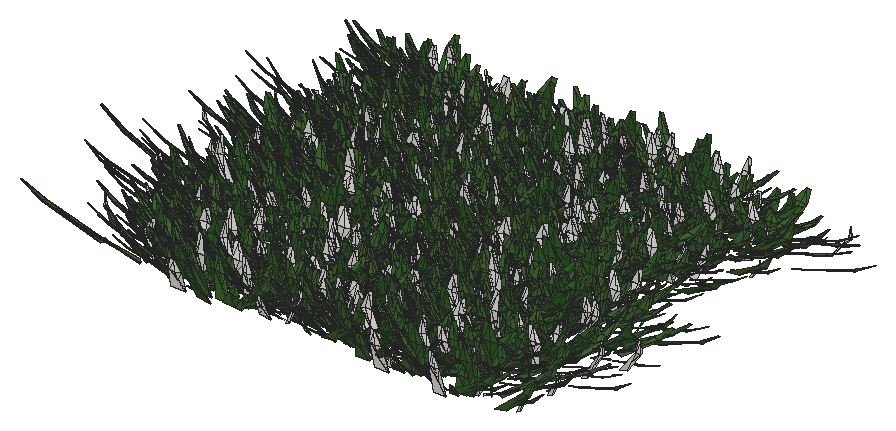
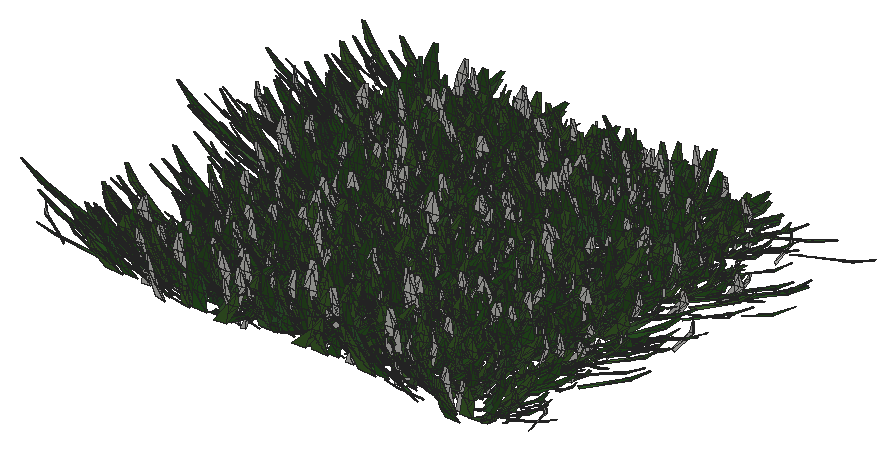
# SketchUp Ruby script. Lengths in inches.
U = 1.inch
M = Sketchup.active_model
def pt(a) = Geom::Point3d.new(a.map { |v| v * U })
def face(e, loops, mat)
  f = e.add_face(loops[0].map { |a| pt(a) })
  loops[1..].each { |l| e.add_face(l.map { |a| pt(a) }).erase! }
  f.material = f.back_material = mat if mat
  f
end
# faces: each face lists its corners as indices into pts; further lists are holes
def faces(e, pts, list, mat = nil) = list.each { |f| face(e, (f[0].is_a?(Array) ? f : [f]).map { |l| l.map { |i| pts[i] } }, mat) }
# xy, xz, yz: faces in a plane at the given z, y or x. An outline is a flat list of corners, or four numbers for a rectangle; further outlines are holes
def ring(l) = l.size == 4 ? [[l[0], l[1]], [l[2], l[1]], [l[2], l[3]], [l[0], l[3]]] : l.each_slice(2).to_a
def flat(e, list, mat, &to3) = list.each { |f| face(e, (f[0].is_a?(Array) ? f : [f]).map { |l| ring(l).map { |u, v| to3.(u, v) } }, mat) }
def xy(e, z, list, mat = nil) = flat(e, list, mat) { |x, y| [x, y, z] }
def xz(e, y, list, mat = nil) = flat(e, list, mat) { |x, z| [x, y, z] }
def yz(e, x, list, mat = nil) = flat(e, list, mat) { |y, z| [x, y, z] }
def lines(e, pts, list) = list.each { |a, b| e.add_line(pt(pts[a]), pt(pts[b])) }
# prism: a flat outline (further loops are holes) pulled along v
def prism(e, loops, v, mat = nil)
  f = face(e, loops, mat); d = Geom::Vector3d.new(v.map { |x| x * U })
  f.pushpull(f.normal.samedirection?(d) ? d.length : -d.length)
end
def box(e, o, s, mat = nil) = prism(e, [[o, [o[0] + s[0], o[1], o[2]], [o[0] + s[0], o[1] + s[1], o[2]], [o[0], o[1] + s[1], o[2]]]], [0, 0, s[2]], mat)
def at(x, y, z, deg = 0) = Geom::Transformation.translation(pt([x, y, z])) * Geom::Transformation.rotation(ORIGIN, Z_AXIS, deg.degrees)
def axes(o, x, y, z) = Geom::Transformation.new([*x, 0, *y, 0, *z, 0, *pt(o).to_a, 1])
def part(name) = M.definitions.add(name)
# library, detail: a bought-in or finely detailed component or shape, given as its bounding box
def library(name, o, s) = part(name).tap { |d| box(d.entities, o, s) }
def detail(e, o, s) = box(e.add_group.entities, o, s)
def put(e, d, t, mat = nil) = e.add_instance(d, t).tap { |i| i.material = mat if mat }
def group(e, t, mat = nil) = e.add_group.tap { |g| g.transformation = t; g.material = mat if mat }.entities
root = M.entities
M.materials.add("Material10").color = [48, 100, 38]
M.materials.add("Material3").color = [68, 110, 58]
M.materials.add("Material4").color = [48, 90, 38]
M.materials.add("Material5").color = [68, 110, 48]
M.materials.add("Material6").color = [48, 90, 48]
M.materials.add("Material7").color = [58, 110, 58]
M.materials.add("Material8").color = [58, 90, 38]
M.materials.add("Material9").color = [68, 100, 58]
c1 = part("grass00")
p = [[-0.6875,0.15,0],[-0.56,0.08,5.52],[-0.04,0.03,2.76],[0.48,-0.02,0],[0.35,-0.02,5.52],[-0.1,-0.14,5.52],
  [-0.12,0.65,8.37],[-0.42,0.65,8.37]]
faces(c1.entities,p,[[0,1,2,3],[3,2,4],[1,5,2],[5,4,2],[1,6,5],[4,5,6],[7,6,1]])
c2 = part("Group16\#1")
put(c2.entities,c1,axes([1.44,-0.61,-0.01],[0.05352,0.12609,0],[-0.10704,0.04543,0.07239],[0.06664,-0.02828,0.11628]),"Material6")
put(c2.entities,c1,axes([0.76,-0.15,-0.01],[0.04676,0.24062,0],[-0.23162,0.04501,0.06642],[0.0652,-0.01267,0.23595]),"Material3")
put(c2.entities,c1,axes([0.79,0.01,-0.01],[-0.00606,0.34651,0],[-0.34381,-0.00602,0.0432],[0.04319,0.00076,0.34386]))
put(c2.entities,c1,axes([1,0.23,-0.01],[-0.07192,0.31144,0],[-0.28722,-0.06632,0.1236],[0.12043,0.02781,0.29478]),"Material5")
put(c2.entities,c1,axes([1.66,0.77,-0.01],[-0.13828,0.29651,0],[-0.21551,-0.1005,0.22471],[0.20365,0.09498,0.23779]),"Material10")
put(c2.entities,c1,axes([0.6875,0.52,-0.01],[-0.18126,0.24051,0],[-0.22746,-0.17142,0.09788],[0.07817,0.05891,0.28481]),"Material5")
put(c2.entities,c1,axes([0.68,0.78,-0.01],[-0.215,0.18688,0],[-0.12385,-0.14248,0.21334],[0.13995,0.16101,0.18878]),"Material3")
put(c2.entities,c1,axes([0.56,1,-0.01],[-0.13756,0.07624,0],[-0.06159,-0.11112,0.0927],[0.04494,0.08108,0.12705]),"Material5")
put(c2.entities,c1,axes([0.2,0.64,-0.01],[-0.23729,0.07254,0],[-0.05711,-0.18681,0.153],[0.04473,0.14632,0.19535]),"Material10")
put(c2.entities,c1,axes([0.0625,0.72,-0.01],[-0.28874,0.02525,0],[-0.02179,-0.24916,0.14647],[0.01276,0.14591,0.25012]),"Material3")
put(c2.entities,c1,axes([-0.08,0.62,-0.01],[-0.34089,-0.04187,0],[0.03255,-0.26504,0.216],[-0.02633,0.21439,0.26703]),"Material10")
put(c2.entities,c1,axes([-0.34,0.98,-0.01],[-0.14314,-0.0493,0],[0.04397,-0.12769,0.06843],[-0.02228,0.0647,0.13505]),"Material10")
put(c2.entities,c1,axes([-0.87,1.45,-0.01],[-0.23488,-0.14114,0],[0.13761,-0.22901,0.06087],[-0.03135,0.05217,0.26717]))
put(c2.entities,c1,axes([-0.72,0.77,-0.01],[-0.14208,-0.13251,0],[0.07209,-0.0773,0.16301],[-0.11118,0.11922,0.1057]),"Material10")
put(c2.entities,c1,axes([-0.62,0.43,-0.01],[-0.14845,-0.21203,0],[0.18654,-0.13061,0.12304],[-0.10079,0.07057,0.22772]),"Material3")
put(c2.entities,c1,axes([-0.68,0.29,-0.01],[-0.13639,-0.32136,0],[0.31723,-0.13464,0.05579],[-0.05136,0.0218,0.34462]),"Material4")
put(c2.entities,c1,axes([-0.64,0.125,-0.01],[-0.0458,-0.23569,0],[0.22124,-0.043,0.08276],[-0.08124,0.01579,0.22538]),"Material7")
put(c2.entities,c1,axes([-1.6,-0.03,-0.01],[0.00576,-0.32897,0],[0.27526,0.00482,0.18018],[-0.18015,-0.00315,0.2753]),"Material5")
put(c2.entities,c1,axes([-1.36,-0.31,-0.01],[0.05718,-0.24765,0],[0.18172,0.04196,0.17267],[-0.16825,-0.03885,0.1865]),"Material10")
put(c2.entities,c1,axes([-1.54,-0.72,-0.01],[0.06537,-0.14017,0],[0.13555,0.06321,0.03939],[-0.0357,-0.01665,0.14956]))
put(c2.entities,c1,axes([-1.19,-0.9,-0.01],[0.09597,-0.12735,0],[0.11214,0.08451,0.07557],[-0.06035,-0.04548,0.14042]),"Material9")
put(c2.entities,c1,axes([-0.47,-0.54,-0.01],[0.11588,-0.10072,0],[0.0618,0.0711,0.12124],[-0.07953,-0.0915,0.0942]))
put(c2.entities,c1,axes([-0.47,-0.84,-0.01],[0.11927,-0.0661,0],[0.06603,0.11913,0.00646],[-0.00313,-0.00565,0.13621]),"Material5")
put(c2.entities,c1,axes([-0.38,-1.24,-0.01],[0.28037,-0.08571,0],[0.0618,0.20215,0.20315],[-0.05939,-0.19428,0.21139]),"Material9")
put(c2.entities,c1,axes([-0.06,-0.66,-0.01],[0.22719,-0.01987,0],[0.01247,0.14255,0.17758],[-0.01547,-0.17691,0.1431]),"Material8")
put(c2.entities,c1,axes([0.11,-0.89,-0.01],[0.14882,0.01828,0],[-0.01058,0.08611,0.12229],[0.01491,-0.12138,0.08676]),"Material6")
put(c2.entities,c1,axes([0.25,-0.72,-0.01],[0.20481,0.07053,0],[-0.06206,0.18022,0.10291],[0.03351,-0.0973,0.1906]),"Material6")
put(c2.entities,c1,axes([0.85,-1.42,-0.01],[0.16481,0.09904,0],[-0.09472,0.15762,0.05616],[0.02893,-0.04814,0.18389]),"Material5")
put(c2.entities,c1,axes([1.01,-1.09,-0.01],[0.21858,0.20385,0],[-0.17495,0.1876,0.15339],[0.10462,-0.11218,0.25652]),"Material10")
put(c2.entities,c1,axes([1.01,-0.71,-0.01],[0.08733,0.12473,0],[-0.06445,0.04512,0.13037],[0.1068,-0.07477,0.07867]),"Material6")
c3 = part("Group15\#1")
put(c3.entities,c2,at(0,0,0))
c4 = part("3darcstudiotree_grass00\#1")
put(c4.entities,c3,at(0,0,0))
put(root,c4,axes([124.42,82.5,7.6],[1.41495,1.18383,0],[-3.49756,0.26127,-0.01522],[-0.0888,0.00663,1.38916]))
put(root,c4,axes([126.49,54.95,7.6],[-4.73179,-0.12886,0],[0.46967,-1.07792,-0.0047],[0.00279,-0.0064,1.4854]))
put(root,c4,axes([124.78,64.93,7.6],[0.18591,1.26274,0],[-5.04075,0.04638,-0.03073],[-0.14495,0.00133,1.48809]))
put(root,c4,axes([126.5625,74.74,7.6],[-4.30621,-0.01829,0],[0.08217,-1.20899,-0.03595],[0.00336,-0.04947,1.66434]))
put(root,c4,axes([126.89,66.41,7.6],[-3.87854,-0.40989,0],[1.77421,-1.04926,-0.0473],[0.09277,-0.05486,1.43445]))
put(root,c4,axes([124.91,54.12,7.6],[4.45359,0.5299,0],[-1.68792,0.88663,-0.01473],[-0.03849,0.02022,1.49308]))
put(root,c4,axes([126.65,57.24,7.6],[-4.3672,0.54864,0],[-1.80768,-0.89932,-0.0516],[-0.17927,-0.08919,1.94674]))
put(root,c4,axes([127.23,59.97,7.6],[-4.20222,0.09704,0],[-0.34915,-0.94494,-0.04806],[-0.02957,-0.08003,1.58689]))
put(root,c4,axes([126.96,73.125,7.6],[2.2244,-0.73123,0],[4.08618,0.77689,-0.04371],[0.15259,0.02901,1.40723]))
put(root,c4,axes([128.02,79.75,7.6],[-4.09129,-0.53085,0],[1.96428,-0.94617,-0.02416],[0.06052,-0.02915,1.4491]))
put(root,c4,axes([128.07,78.01,7.6],[-3.27232,-0.38033,0],[1.61038,-0.86597,-0.04575],[0.12951,-0.06964,1.60296]))
put(root,c4,axes([126.875,69.46,7.6],[1.34498,0.85271,0],[-3.61197,0.35607,-0.04901],[-0.30956,0.03052,1.64754]))
put(root,c4,axes([128.14,51.875,7.6],[-3.74465,0.10964,0],[-0.44388,-0.94751,-0.03745],[-0.02749,-0.05868,1.50509]))
put(root,c4,axes([126.73,47.91,7.6],[0.55868,1.18187,0],[-4.38906,0.12967,-0.00527],[-0.02848,0.00084,1.50433]))
put(root,c4,axes([127.38,81.63,7.6],[3.92571,-0.06568,0],[0.27031,1.00981,-0.02393],[0.00951,0.03553,1.50627]))
put(root,c4,axes([127.24,67.3,7.6],[4.1204,0.14772,0],[-0.55424,0.96623,-0.02285],[-0.01788,0.03117,1.34478]))
put(root,c4,axes([128.85,44.9375,7.6],[-4.54837,0.61423,0],[-2.27056,-1.05085,-0.03525],[-0.07342,-0.03398,1.3087]))
put(root,c4,axes([129.04,49.74,7.6],[1.35556,-1.09662,0],[3.48641,0.26935,-0.00928],[0.07297,0.00564,1.87692]))
put(root,c4,axes([127.76,58.58,7.6],[4.58081,0.57203,0],[-2.05118,1.02662,-0.04234],[-0.09467,0.04738,1.4356]))
put(root,c4,axes([128.33,72.32,7.6],[4.09069,0.39107,0],[-1.49345,0.97637,-0.02441],[-0.06576,0.04299,1.97124]))
put(root,c4,axes([128.3,70.53,7.6],[4.67312,0.46375,0],[-1.55175,0.97728,-0.04113],[-0.07938,0.05,1.37498]))
put(root,c4,axes([128.86,76.31,7.6],[1.74991,0.88126,0],[-3.81182,0.47307,-0.01001],[-0.04959,0.00615,1.4706]))
put(root,c4,axes([130.88,63.98,7.6],[-4.64971,-0.14285,0],[0.57946,-1.17887,-0.04768],[0.02933,-0.05967,1.49744]))
put(root,c4,axes([129.26,53.72,7.6],[0.96395,1.06005,0],[-4.81113,0.27344,-0.06457],[-0.29518,0.01678,1.44574]))
put(root,c4,axes([130.38,46.22,7.6],[3.00205,-0.85659,0],[3.63036,0.7952,-0.04981],[0.2075,0.04545,1.67091]))
put(root,c4,axes([129.4,62.67,7.6],[3.43592,0.73211,0],[-2.51322,0.73719,-0.00613],[-0.02752,0.00807,1.67562]))
put(root,c4,axes([130.35,50.32,7.6],[1.74385,0.8383,0],[-3.77239,0.49046,-0.03549],[-0.18091,0.02352,1.52707]))
put(root,c4,axes([130.11,61.6,7.6],[1.69559,1.05532,0],[-4.4836,0.45024,-0.00669],[-0.03988,0.004,1.94122]))
put(root,c4,axes([133.36,44.27,7.6],[-2.1334,-0.73078,0],[3.43772,-0.62725,-0.00015],[0.00089,-0.00016,1.94435]))
put(root,c4,axes([133.04,61.22,7.6],[-0.05318,-0.92593,0],[5.00241,-0.01796,-0.06189],[0.33029,-0.00119,1.66883]))
put(root,c4,axes([133.4,80.03,7.6],[-3.23712,-0.63399,0],[2.66966,-0.85194,-0.04081],[0.13619,-0.04346,1.46417]))
put(root,c4,axes([133.35,73.37,7.6],[-4.03858,-0.16836,0],[0.61274,-0.91864,-0.01602],[0.01597,-0.02395,1.41148]))
put(root,c4,axes([134.01,81.37,7.6],[-0.4686,-0.94109,0],[4.875,-0.15171,-0.05859],[0.34766,-0.01082,1.83593]))
put(root,c4,axes([134.38,66.01,7.6],[-4.976,0.12548,0],[-0.39366,-0.97566,-0.00469],[-0.00376,-0.00932,1.96044]))
put(root,c4,axes([134.65,67.66,7.6],[-3.93213,0.25374,0],[-1.01516,-0.98322,-0.03018],[-0.05893,-0.05707,1.98332]))
put(root,c4,axes([135.21,77.64,7.6],[-3.81287,-0.39073,0],[1.76767,-1.0781,-0.01809],[0.03493,-0.0213,1.4829]))
put(root,c4,axes([134.63,76.28,7.6],[1.16902,-1.01976,0],[4.12301,0.2954,-0.03571],[0.25113,0.01799,1.9611]))
put(root,c4,axes([134.76,46.48,7.6],[-3.57612,0.46,0],[-1.68045,-0.8165,-0.01759],[-0.06739,-0.03274,1.92222]))
put(root,c4,axes([134.52,55.21,7.6],[2.75353,-0.91552,0],[4.13951,0.77813,-0.05965],[0.29097,0.05469,1.97549]))
put(root,c4,axes([133.67,70.53,7.6],[4.41787,0.20597,0],[-0.82473,1.10563,-0.00417],[-0.0051,0.00683,1.87295]))
put(root,c4,axes([135.39,56.4,7.6],[-0.77256,-1.09422,0],[3.72876,-0.16454,-0.01992],[0.13289,-0.00586,1.60321]))
put(root,c4,axes([133.66,52.31,7.6],[4.90123,0.13236,0],[-0.55386,1.28181,-0.03307],[-0.01756,0.04064,1.59331]))
put(root,c4,axes([134.13,63.08,7.6],[0.63816,1.22279,0],[-3.70201,0.12075,-0.03746],[-0.26805,0.00874,1.68385]))
put(root,c4,axes([134.88,50.37,7.6],[-3.38877,0.51557,0],[-2.38455,-0.97958,-0.01391],[-0.04361,-0.01791,1.7292]))
put(root,c4,axes([135.11,53.53,7.6],[2.69835,-0.96968,0],[3.12111,0.54282,-0.02795],[0.17981,0.03127,1.86246]))
put(root,c4,axes([134.76,69.01,7.6],[-2.15572,1.01928,0],[-4.46043,-0.5896,-0.01892],[-0.07769,-0.01027,1.46501]))
put(root,c4,axes([136.66,75.07,7.6],[-3.178,-0.72198,0],[3.25819,-0.89636,-0.02206],[0.07961,-0.0219,1.62457]))
put(root,c4,axes([135,58.75,7.6],[-2.01821,1.07087,0],[-4.04462,-0.47641,-0.00165],[-0.00796,-0.00094,1.48801]))
put(root,c4,axes([136.75,47.43,7.6],[-5.04293,-0.12413,0],[0.46059,-1.16949,-0.00134],[0.0006,-0.00152,1.33719]))
put(root,c4,axes([134.69,72.55,7.6],[1.81913,1.13072,0],[-4.24624,0.42697,-0.0015],[-0.00751,0.00076,1.54039]))
put(root,c4,axes([136.29,49.35,7.6],[2.93485,-0.98597,0],[3.93521,0.7321,-0.05496],[0.20354,0.03787,1.41537]))
put(root,c4,axes([136.5,59.75,7.6],[0.69977,0.95429,0],[-4.68091,0.21453,-0.00804],[-0.04724,0.00217,1.77733]))
put(root,c4,axes([136.77,64.87,7.6],[2.05265,1.08844,0],[-3.86298,0.45532,-0.03917],[-0.23834,0.02809,1.79585]))
put(root,c4,axes([139.52,47.65,7.6],[-1.12524,-0.96886,0],[3.74948,-0.27217,-0.00444],[0.03259,-0.00237,1.86591]))
put(root,c4,axes([138.9,61.27,7.6],[1.4605,-0.95002,0],[3.8779,0.3726,-0.03841],[0.24153,0.02321,1.74904]))
put(root,c4,axes([139.41,67.22,7.6],[-2.14754,-0.73736,0],[3.76224,-0.68483,-0.06067],[0.30518,-0.05555,1.80988]))
put(root,c4,axes([139.29,50.73,7.6],[-3.33972,0.41247,0],[-1.92358,-0.97344,-0.03032],[-0.07425,-0.03758,1.50108]))
put(root,c4,axes([139.27,72.47,7.6],[3.71164,-0.61185,0],[2.58785,0.98115,-0.02666],[0.07433,0.02818,1.48784]))
put(root,c4,axes([140.375,81.02,7.6],[0.28174,-1.01382,0],[4.36389,0.07579,-0.0172],[0.10528,0.00183,1.67763]))
put(root,c4,axes([139.93,45.37,7.6],[-2.86097,0.86073,0],[-3.01972,-0.62732,-0.04997],[-0.22994,-0.04777,1.46822]))
put(root,c4,axes([141.125,71.12,7.6],[-4.12883,-0.65967,0],[2.58219,-1.01011,-0.05584],[0.19452,-0.07609,1.93872]))
put(root,c4,axes([139.63,49.74,7.6],[-0.2845,0.94758,0],[-4.0362,-0.07574,-0.02554],[-0.16533,-0.0031,1.64241]))
put(root,c4,axes([141.5625,53.39,7.6],[-4.76231,0.21357,0],[-0.8747,-1.21904,-0.00093],[-0.00084,-0.00117,1.58752]))
put(root,c4,axes([140.26,46.6,7.6],[4.17112,0.04454,0],[-0.19892,1.16431,-0.01987],[-0.00428,0.02505,1.47043]))
put(root,c4,axes([140.29,55.31,7.6],[4.56851,-0.0546,0],[0.17436,0.91177,-0.03217],[0.01167,0.06102,1.73328]))
put(root,c4,axes([140.5,56.74,7.6],[4.23657,-0.2376,0],[0.80233,0.89415,-0.00297],[0.00478,0.00533,1.68702]))
put(root,c4,axes([142.35,78.12,7.6],[-3.12199,-0.46434,0],[2.64637,-1.11204,-0.00321],[0.00751,-0.00316,1.48019]))
put(root,c4,axes([141.49,73.17,7.6],[-3.87477,0.75183,0],[-2.84001,-0.9148,-0.03049],[-0.11215,-0.03613,1.73706]))
put(root,c4,axes([140.73,63.55,7.6],[3.58042,0.48605,0],[-1.82681,0.84106,-0.03457],[-0.13256,0.06103,1.92264]))
put(root,c4,axes([141.78,76.84,7.6],[2.19573,-0.79563,0],[3.28578,0.56674,-0.0362],[0.23043,0.03975,1.92943]))
put(root,c4,axes([141.35,52.67,7.6],[-1.60767,1.01804,0],[-4.53552,-0.44765,-0.02576],[-0.12044,-0.01189,1.53201]))
put(root,c4,axes([141.4375,58.17,7.6],[4.66104,-0.01291,0],[0.04336,0.97863,-0.01976],[0.00122,0.02762,1.36845]))
put(root,c4,axes([141.69,65.9375,7.6],[2.73136,0.67519,0],[-2.53096,0.63991,-0.02576],[-0.15171,0.03836,1.88472]))
put(root,c4,axes([141.8,68.65,7.6],[4.8227,0.33397,0],[-1.37587,1.24178,-0.02222],[-0.03562,0.03215,1.93436]))
put(root,c4,axes([142.17,79.72,7.6],[2.66703,0.73786,0],[-3.13866,0.70905,-0.0306],[-0.16013,0.03617,1.86488]))
put(root,c4,axes([143.03,59.4375,7.6],[-2.52556,0.85651,0],[-3.11909,-0.57482,-0.0238],[-0.1265,-0.02331,1.59896]))
put(root,c4,axes([142.32,75.5625,7.6],[1.56451,1.00298,0],[-4.78607,0.4666,-0.01645],[-0.08409,0.0082,1.76201]))
put(root,c4,axes([142.62,65.03,7.6],[1.42494,0.93436,0],[-3.83119,0.36517,-0.01397],[-0.07753,0.00739,1.52193]))
put(root,c4,axes([145.43,46.8125,7.6],[-3.14311,-1.03345,0],[3.53925,-0.67276,-0.02],[0.10195,-0.01938,1.779]))
put(root,c4,axes([145.19,47.78,7.6],[-0.38253,-1.25706,0],[5.07372,-0.0965,-0.05882],[0.29497,-0.00561,1.5994]))
put(root,c4,axes([145.6,55.89,7.6],[-3.9211,-0.27648,0],[1.04934,-0.93013,-0.015],[0.02202,-0.01952,1.30652]))
put(root,c4,axes([144.72,78.3125,7.6],[-0.95414,1.15068,0],[-4.04773,-0.20977,-0.02464],[-0.16776,-0.00869,1.79662]))
put(root,c4,axes([145.44,49.37,7.6],[-3.41535,0.94101,0],[-3.19182,-0.72403,-0.0082],[-0.03901,-0.00885,1.73071]))
put(root,c4,axes([145.14,77.02,7.6],[-0.26244,0.97433,0],[-4.33641,-0.073,-0.04305],[-0.28268,-0.00476,1.78778]))
put(root,c4,axes([146.28,65.52,7.6],[-4.734,0.44651,0],[-1.80443,-1.19569,-0.03096],[-0.06152,-0.04076,1.79846]))
put(root,c4,axes([146.89,54.35,7.6],[-3.54413,-0.35283,0],[1.88693,-1.18461,-0.01803],[0.03799,-0.02385,1.81493]))
put(root,c4,axes([145.7,62.8125,7.6],[-1.93923,0.80033,0],[-4.36084,-0.6604,-0.05645],[-0.30002,-0.04543,1.97994]))
put(root,c4,axes([147.17,74.11,7.6],[-1.73824,-0.83269,0],[3.93121,-0.5129,-0.00435],[0.02089,-0.00273,1.50222]))
put(root,c4,axes([145.54,61.65,7.6],[3.26249,0.60372,0],[-2.60827,0.88094,-0.05487],[-0.17274,0.05834,1.44987]))
put(root,c4,axes([145.65,79.57,7.6],[0.73959,1.18717,0],[-3.65318,0.14224,-0.00889],[-0.05312,0.00207,1.39664]))
put(root,c4,axes([146.51,81.39,7.6],[2.83501,-0.87969,0],[3.07253,0.61887,-0.02709],[0.15503,0.03123,1.8123]))
put(root,c4,axes([145.54,70.86,7.6],[4.22317,0.50582,0],[-2.02967,1.05913,-0.04599],[-0.0924,0.04822,1.36526]))
put(root,c4,axes([147.79,74.82,7.6],[-3.49567,-0.41418,0],[1.84622,-0.97387,-0.03887],[0.09057,-0.04778,1.46596]))
put(root,c4,axes([146.88,60.14,7.6],[3.68446,-0.69974,0],[2.40562,0.79167,-0.03309],[0.11614,0.03822,1.44206]))
put(root,c4,axes([148.27,67.36,7.6],[-3.25249,-0.4237,0],[1.99269,-0.95605,-0.0201],[0.0448,-0.0215,1.30027]))
put(root,c4,axes([148.47,52.24,7.6],[-3.91695,-0.76183,0],[3.11851,-1.00211,-0.06227],[0.16525,-0.0531,1.37168]))
put(root,c4,axes([146.54,71.95,7.6],[1.52552,1.07764,0],[-3.72178,0.32929,-0.0171],[-0.12069,0.01068,1.84743]))
put(root,c4,axes([147.23,45.08,7.6],[-0.98833,1.19917,0],[-3.8776,-0.19974,-0.03296],[-0.18407,-0.00948,1.411]))
put(root,c4,axes([147.41,58.375,7.6],[-1.74933,1.03948,0],[-3.53507,-0.37182,-0.02216],[-0.14167,-0.0149,1.66252]))
put(root,c4,axes([148.53,68.58,7.6],[3.35043,-0.75633,0],[2.9183,0.80798,-0.04418],[0.18264,0.05057,1.67893]))
put(root,c4,axes([148.26,50.58,7.6],[-0.82221,1.07388,0],[-4.85232,-0.2322,-0.01652],[-0.07909,-0.00378,1.50529]))
put(root,c4,axes([148.47,64.45,7.6],[4.38567,-0.08429,0],[0.3564,1.15903,-0.03486],[0.01549,0.05039,1.68524]))
put(root,c4,axes([148.91,56.75,7.6],[4.19452,0.71588,0],[-2.43274,0.89088,-0.02215],[-0.08774,0.03213,1.8946]))
put(root,c4,axes([150.94,67.6,7.6],[0.50446,-1.28497,0],[4.75288,0.11662,-0.05803],[0.25331,0.00622,1.30918]))
put(root,c4,axes([151.8125,70.74,7.6],[-3.01986,-0.89757,0],[3.46122,-0.72782,-0.04595],[0.21791,-0.04582,1.75181]))
put(root,c4,axes([151.3,72.57,7.6],[2.394,-0.81419,0],[3.9298,0.72218,-0.0227],[0.09655,0.01774,1.60931]))
put(root,c4,axes([152.08,54,7.6],[-4.0317,-0.25141,0],[0.95302,-0.95517,-0.04204],[0.06722,-0.06737,1.62585]))
put(root,c4,axes([151.7,44.71,7.6],[-4.15536,0.77828,0],[-2.7986,-0.93389,-0.03017],[-0.1071,-0.03574,1.72726]))
put(root,c4,axes([150.92,69.35,7.6],[1.24349,0.95069,0],[-4.25943,0.34821,-0.05705],[-0.29582,0.02418,1.52794]))
put(root,c4,axes([152.77,77.22,7.6],[-3.8617,-0.01302,0],[0.05631,-1.04356,-0.03579],[0.00298,-0.05513,1.60809]))
put(root,c4,axes([152.11,61.51,7.6],[-3.40266,0.70782,0],[-3.16523,-0.95101,-0.01948],[-0.07283,-0.02188,1.80807]))
put(root,c4,axes([152.39,81.72,7.6],[-3.32672,0.63857,0],[-2.74378,-0.89337,-0.05552],[-0.19615,-0.06387,1.63365]))
put(root,c4,axes([151.14,74.65,7.6],[1.64031,0.90171,0],[-3.63622,0.41342,-0.00419],[-0.02649,0.00301,1.73548]))
put(root,c4,axes([152.34,59.77,7.6],[3.62794,-0.3827,0],[1.97795,1.17191,-0.0407],[0.07531,0.04462,1.51351]))
put(root,c4,axes([151.53,46.87,7.6],[3.52874,0.5715,0],[-2.37881,0.918,-0.01048],[-0.03241,0.01251,1.55517]))
put(root,c4,axes([153.88,58.6,7.6],[-4.67502,-0.56796,0],[2.06884,-1.06432,-0.01545],[0.04157,-0.02139,1.8215]))
put(root,c4,axes([151.54,77.84,7.6],[2.90908,1.00895,0],[-3.39125,0.61112,-0.01552],[-0.0694,0.01251,1.43977]))
put(root,c4,axes([152.47,55.37,7.6],[0.16489,0.91256,0],[-4.05383,0.04578,-0.0329],[-0.25692,0.0029,1.98251]))
put(root,c4,axes([152.43,49.89,7.6],[-0.75214,1.19237,0],[-4.74693,-0.18715,-0.03641],[-0.174,-0.00686,1.45326]))
put(root,c4,axes([152.53,73.375,7.6],[4.69551,-0.08423,0],[0.3605,1.25607,-0.01186],[0.0041,0.0143,1.52253]))
put(root,c4,axes([153.4,82.24,7.6],[2.38234,-0.95226,0],[3.20328,0.50086,-0.0272],[0.17769,0.02778,1.81972]))
put(root,c4,axes([152.9,50.46,7.6],[-1.46228,1.23307,0],[-3.47122,-0.25728,-0.00114],[-0.00907,-0.00067,1.86907]))
put(root,c4,axes([152.39,56.47,7.6],[1.47006,1.1325,0],[-4.40979,0.35776,-0.01715],[-0.07948,0.00645,1.41194]))
put(root,c4,axes([153.58,62.99,7.6],[-2.07415,0.83506,0],[-3.95028,-0.61324,-0.02009],[-0.09896,-0.01536,1.68525]))
put(root,c4,axes([154.46,64.9,7.6],[-1.18382,1.15457,0],[-4.70826,-0.30172,-0.05431],[-0.29177,-0.0187,1.6847]))
put(root,c4,axes([154.88,79.8,7.6],[-3.28461,0.98923,0],[-3.37325,-0.70003,-0.00469],[-0.02101,-0.00436,1.59556]))
put(root,c4,axes([154.32,66.25,7.6],[2.88148,0.64126,0],[-3.12484,0.87758,-0.03405],[-0.12784,0.0359,1.65877]))
put(root,c4,axes([154.61,52.33,7.6],[3.07935,0.60729,0],[-3.11371,0.98678,-0.06164],[-0.16424,0.05205,1.3518]))
put(root,c4,axes([154.98,47.7,7.6],[0.52678,1.06322,0],[-4.94177,0.15303,-0.03401],[-0.15238,0.00472,1.40523]))
put(root,c4,axes([157.28,69.64,7.6],[1.39418,-0.83958,0],[3.77377,0.39166,-0.03248],[0.18939,0.01966,1.61223]))
put(root,c4,axes([157.7,59.43,7.6],[-4.00371,0.05544,0],[-0.23957,-1.08136,-0.04105],[-0.01536,-0.06935,1.83253]))
put(root,c4,axes([156.8,70.97,7.6],[-0.74123,1.26839,0],[-3.97906,-0.14533,-0.03578],[-0.18887,-0.0069,1.34076]))
put(root,c4,axes([157.72,44.3,7.6],[-3.45273,0.48202,0],[-2.12645,-0.95198,-0.05669],[-0.18901,-0.08462,1.86391]))
put(root,c4,axes([158.375,52.33,7.6],[-2.58874,-0.9071,0],[3.15855,-0.56338,-0.04134],[0.26965,-0.0481,1.943]))
put(root,c4,axes([157.58,48.4,7.6],[-3.19228,0.66883,0],[-3.28024,-0.97852,-0.01682],[-0.06095,-0.01818,1.80026]))
put(root,c4,axes([157.96,74.875,7.6],[-3.68677,0.78294,0],[-2.37097,-0.69779,-0.00331],[-0.01382,-0.00407,1.47415]))
put(root,c4,axes([158.45,51.41,7.6],[2.79001,-0.91126,0],[3.28074,0.62779,-0.00025],[0.00114,0.00022,1.45509]))
put(root,c4,axes([158.27,61.41,7.6],[3.11012,-0.98955,0],[3.48139,0.68387,-0.04001],[0.20872,0.041,1.83572]))
put(root,c4,axes([157.52,57.07,7.6],[4.49844,0.3136,0],[-1.0523,0.94343,-0.03867],[-0.07449,0.06678,1.75619]))
put(root,c4,axes([157.89,76.65,7.6],[0.32984,1.08986,0],[-4.10586,0.07766,-0.04286],[-0.23653,0.00447,1.42447]))
put(root,c4,axes([159.67,55.67,7.6],[-3.31262,-0.80999,0],[3.0672,-0.784,-0.0483],[0.19534,-0.04993,1.58573]))
put(root,c4,axes([158.79,78.08,7.6],[3.83987,-0.74679,0],[3.08152,0.9903,-0.05588],[0.18273,0.05872,1.67045]))
put(root,c4,axes([160.3,80.8,7.6],[-1.00327,-1.08198,0],[4.89707,-0.2838,-0.01344],[0.05958,-0.00345,1.42931]))
